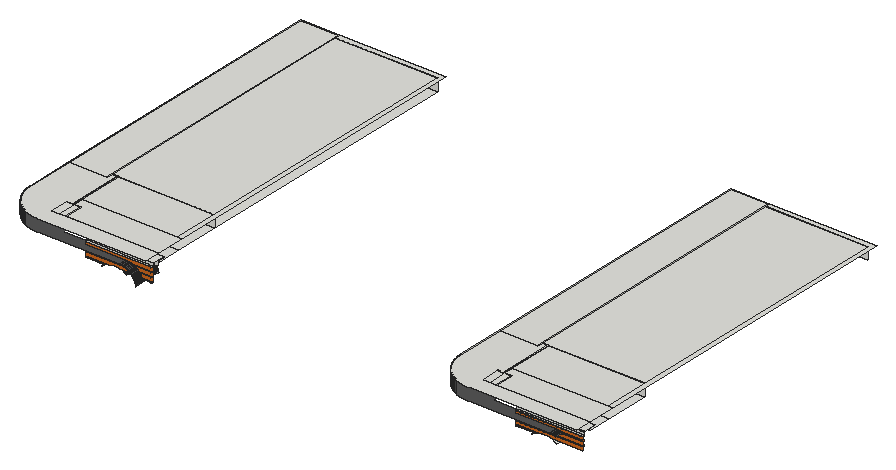
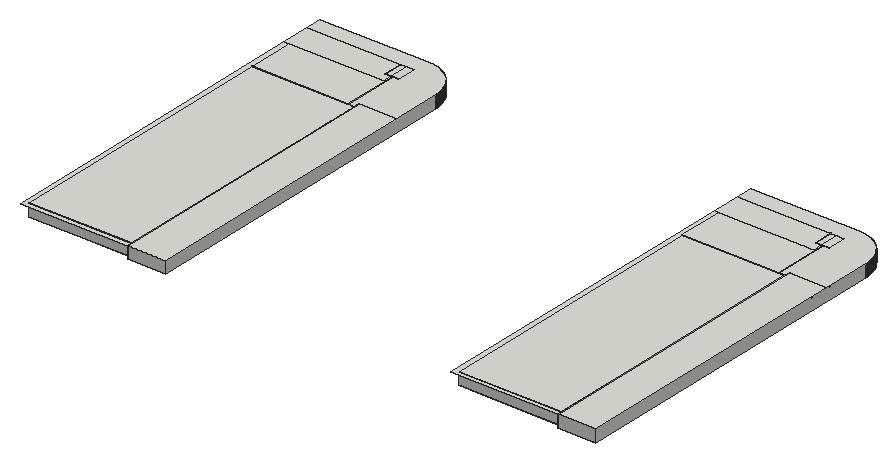
# SketchUp Ruby script. Lengths in inches.
U = 1.inch
M = Sketchup.active_model
def pt(a) = Geom::Point3d.new(a.map { |v| v * U })
def face(e, loops, mat)
  f = e.add_face(loops[0].map { |a| pt(a) })
  loops[1..].each { |l| e.add_face(l.map { |a| pt(a) }).erase! }
  f.material = f.back_material = mat if mat
  f
end
# faces: each face lists its corners as indices into pts; further lists are holes
def faces(e, pts, list, mat = nil) = list.each { |f| face(e, (f[0].is_a?(Array) ? f : [f]).map { |l| l.map { |i| pts[i] } }, mat) }
# xy, xz, yz: faces in a plane at the given z, y or x. An outline is a flat list of corners, or four numbers for a rectangle; further outlines are holes
def ring(l) = l.size == 4 ? [[l[0], l[1]], [l[2], l[1]], [l[2], l[3]], [l[0], l[3]]] : l.each_slice(2).to_a
def flat(e, list, mat, &to3) = list.each { |f| face(e, (f[0].is_a?(Array) ? f : [f]).map { |l| ring(l).map { |u, v| to3.(u, v) } }, mat) }
def xy(e, z, list, mat = nil) = flat(e, list, mat) { |x, y| [x, y, z] }
def xz(e, y, list, mat = nil) = flat(e, list, mat) { |x, z| [x, y, z] }
def yz(e, x, list, mat = nil) = flat(e, list, mat) { |y, z| [x, y, z] }
def lines(e, pts, list) = list.each { |a, b| e.add_line(pt(pts[a]), pt(pts[b])) }
# prism: a flat outline (further loops are holes) pulled along v
def prism(e, loops, v, mat = nil)
  f = face(e, loops, mat); d = Geom::Vector3d.new(v.map { |x| x * U })
  f.pushpull(f.normal.samedirection?(d) ? d.length : -d.length)
end
def box(e, o, s, mat = nil) = prism(e, [[o, [o[0] + s[0], o[1], o[2]], [o[0] + s[0], o[1] + s[1], o[2]], [o[0], o[1] + s[1], o[2]]]], [0, 0, s[2]], mat)
def at(x, y, z, deg = 0) = Geom::Transformation.translation(pt([x, y, z])) * Geom::Transformation.rotation(ORIGIN, Z_AXIS, deg.degrees)
def axes(o, x, y, z) = Geom::Transformation.new([*x, 0, *y, 0, *z, 0, *pt(o).to_a, 1])
def part(name) = M.definitions.add(name)
# library, detail: a bought-in or finely detailed component or shape, given as its bounding box
def library(name, o, s) = part(name).tap { |d| box(d.entities, o, s) }
def detail(e, o, s) = box(e.add_group.entities, o, s)
def put(e, d, t, mat = nil) = e.add_instance(d, t).tap { |i| i.material = mat if mat }
def group(e, t, mat = nil) = e.add_group.tap { |g| g.transformation = t; g.material = mat if mat }.entities
root = M.entities
M.materials.add("[0041_Chocolate]").color = [210, 105, 30]
M.materials.add("[Color M06]").color = [84, 84, 84]
xy(root,385.02,[[820.52,971.36,850.01,972.36],[877.83,971.36,921.96,972.36],[1476.02,971.36,1505.51,972.36]],"[0041_Chocolate]")
xy(root,386.9375,[[820.52,971.36,854.99,972.36],[872.87,971.36,921.96,972.36],[1476.02,971.36,1510.49,972.36]],"[0041_Chocolate]")
xy(root,391.89,[[820.52,971.36,921.96,972.36],[1476.02,971.36,1577.46,972.36]],"[0041_Chocolate]")
xy(root,393.8125,[[820.52,971.36,921.96,972.36],[1476.02,971.36,1577.46,972.36]],"[0041_Chocolate]")
xy(root,395.26,[[820.52,993.35,899.77,1001.16],[1476.02,993.35,1555.27,1001.16]])
xy(root,398.77,[[820.52,971.36,921.96,972.36],[1476.02,971.36,1577.46,972.36]],"[0041_Chocolate]")
xy(root,400.6875,[[820.52,971.36,921.96,972.36],[1476.02,971.36,1577.46,972.36]],"[0041_Chocolate]")
xy(root,402.64,[[820.52,991.23,881.73,993.35],[1476.02,991.23,1537.23,993.35],[913.34,993.35,916.04,993.35,916.04,1028.46,769.03,1028.46,769.03,1012.23,780.56,1012.23,780.56,996.48,820.52,996.48,820.52,1003.71,913.34,1003.71],[820.52,993.35,913.34,1003.71],[1568.84,993.35,1571.54,993.35,1571.54,1028.46,1424.53,1028.46,1424.53,1012.23,1436.06,1012.23,1436.06,996.48,1476.02,996.48,1476.02,1003.71,1568.84,1003.71],
  [1476.02,993.35,1568.84,1003.71],[759.32,996.48,769.03,1003.71],[769.03,996.48,780.56,1003.71],[1414.82,996.48,1424.53,1003.71],[1424.53,996.48,1436.06,1003.71],
  [759.32,1003.71,769.03,1012.23],[769.03,1003.71,780.56,1012.23],[1414.82,1003.71,1424.53,1012.23],[1424.53,1003.71,1436.06,1012.23],[769.03,1028.46,916.04,1097.28],
  [1424.53,1028.46,1571.54,1097.28],[767.84,1089.96,769.03,1097.28],[1423.34,1089.96,1424.53,1097.28],[759.32,1097.28,767.84,1521.81],[767.84,1097.28,879.04,1521.81],
  [879.04,1097.28,916.04,1521.81],[1414.82,1097.28,1423.34,1521.81],[1423.34,1097.28,1534.54,1521.81]])
xy(root,402.64,[[758.26,958.64,756.78,958.66,755.29,958.72,753.8,958.82,752.32,958.96,750.84,959.13,749.37,959.34,747.9,959.6,746.4375,959.89,744.98,960.22,743.54,960.58,742.11,960.99,740.6875,961.43,739.28,961.91,737.88,962.42,736.49,962.97,735.125,963.5625,733.77,964.1875,732.4375,964.84,731.12,965.54,729.82,966.27,728.54,967.03,727.28,967.82,726.04,968.65,724.83,969.51,723.63,970.4,722.46,971.32,721.32,972.27,720.2,973.26,719.11,974.27,718.04,975.31,717,976.37,715.99,977.47,715.01,978.59,714.06,979.73,713.13,980.9,712.24,982.09,711.38,983.31,710.56,984.55,709.76,985.81,709,987.09,708.27,988.39,707.58,989.71,706.92,991.04,706.3,992.39,705.71,993.76,705.16,995.14,704.64,996.54,704.16,997.95,703.72,999.375,703.32,1000.81,702.95,1002.25,702.62,1003.7,702.33,1005.16,702.08,1006.63,701.86,1008.11,701.6875,1009.58,701.55,1011.07,701.46,1012.55,701.4,1014.04,701.38,1015.53,701.38,1529.04,759.32,1529.04,759.32,996.48,780.56,996.48,780.56,978.84,820.52,978.84,820.52,991.23,881.73,991.23,881.73,958.64],[1413.76,958.64,1412.28,958.66,1410.79,958.72,1409.3,958.82,1407.82,958.96,1406.34,959.13,1404.87,959.34,1403.4,959.6,1401.9375,959.89,1400.48,960.22,1399.04,960.58,1397.61,960.99,1396.1875,961.43,1394.78,961.91,1393.38,962.42,1391.99,962.97,1390.625,963.5625,1389.27,964.1875,1387.9375,964.84,1386.62,965.54,1385.32,966.27,1384.04,967.03,1382.78,967.82,1381.54,968.65,1380.33,969.51,1379.13,970.4,1377.96,971.32,1376.82,972.27,1375.7,973.26,1374.61,974.27,1373.54,975.31,1372.5,976.37,1371.49,977.47,1370.51,978.59,1369.56,979.73,1368.63,980.9,1367.74,982.09,1366.88,983.31,1366.06,984.55,1365.26,985.81,1364.5,987.09,1363.77,988.39,1363.08,989.71,1362.42,991.04,1361.8,992.39,1361.21,993.76,1360.66,995.14,1360.14,996.54,1359.66,997.95,1359.22,999.375,1358.82,1000.81,1358.45,1002.25,1358.12,1003.7,1357.83,1005.16,1357.58,1006.63,1357.36,1008.11,1357.1875,1009.58,1357.05,1011.07,1356.96,1012.55,1356.9,1014.04,1356.88,1015.53,1356.88,1529.04,1414.82,1529.04,1414.82,996.48,1436.06,996.48,1436.06,978.84,1476.02,978.84,1476.02,991.23,1537.23,991.23,1537.23,958.64]],"[Color M06]")
xy(root,405.64,[[820.52,971.36,921.96,972.36],[1476.02,971.36,1577.46,972.36]],"[0041_Chocolate]")
xy(root,411.82,[[820.52,972.36,921.96,993.35],[1476.02,972.36,1577.46,993.35]])
xy(root,421.25,[[758.26,958.64,922.83,958.64,922.83,983.34,759.32,983.34,759.32,1012.23,767.84,1012.23,767.84,1097.28,759.32,1097.28,759.32,1088.75,701.38,1088.75,701.38,1015.53,701.4,1014.04,701.46,1012.55,701.55,1011.07,701.6875,1009.58,701.86,1008.11,702.08,1006.63,702.33,1005.16,702.62,1003.7,702.95,1002.25,703.32,1000.81,703.72,999.375,704.16,997.95,704.64,996.54,705.16,995.14,705.71,993.76,706.3,992.39,706.92,991.04,707.58,989.71,708.27,988.39,709,987.09,709.76,985.81,710.56,984.55,711.38,983.31,712.24,982.09,713.13,980.9,714.06,979.73,715.01,978.59,715.99,977.47,717,976.37,718.04,975.31,719.11,974.27,720.2,973.26,721.32,972.27,722.46,971.32,723.63,970.4,724.83,969.51,726.04,968.65,727.28,967.82,728.54,967.03,729.82,966.27,731.12,965.54,732.4375,964.84,733.77,964.1875,735.125,963.5625,736.49,962.97,737.88,962.42,739.28,961.91,740.6875,961.43,742.11,960.99,743.54,960.58,744.98,960.22,746.4375,959.89,747.9,959.6,749.37,959.34,750.84,959.13,752.32,958.96,753.8,958.82,755.29,958.72,756.78,958.66],[1413.76,958.64,1578.33,958.64,1578.33,983.34,1414.82,983.34,1414.82,1012.23,1423.34,1012.23,1423.34,1097.28,1414.82,1097.28,1414.82,1088.75,1356.88,1088.75,1356.88,1015.53,1356.9,1014.04,1356.96,1012.55,1357.05,1011.07,1357.1875,1009.58,1357.36,1008.11,1357.58,1006.63,1357.83,1005.16,1358.12,1003.7,1358.45,1002.25,1358.82,1000.81,1359.22,999.375,1359.66,997.95,1360.14,996.54,1360.66,995.14,1361.21,993.76,1361.8,992.39,1362.42,991.04,1363.08,989.71,1363.77,988.39,1364.5,987.09,1365.26,985.81,1366.06,984.55,1366.88,983.31,1367.74,982.09,1368.63,980.9,1369.56,979.73,1370.51,978.59,1371.49,977.47,1372.5,976.37,1373.54,975.31,1374.61,974.27,1375.7,973.26,1376.82,972.27,1377.96,971.32,1379.13,970.4,1380.33,969.51,1381.54,968.65,1382.78,967.82,1384.04,967.03,1385.32,966.27,1386.62,965.54,1387.9375,964.84,1389.27,964.1875,1390.625,963.5625,1391.99,962.97,1393.38,962.42,1394.78,961.91,1396.1875,961.43,1397.61,960.99,1399.04,960.58,1400.48,960.22,1401.9375,959.89,1403.4,959.6,1404.87,959.34,1406.34,959.13,1407.82,958.96,1409.3,958.82,1410.79,958.72,1412.28,958.66],[759.32,983.34,770.9,1012.23],[770.9,983.34,780.56,1012.23],[780.56,983.34,922.83,983.34,922.83,1027.17,770.9,1027.17,770.9,1012.23,780.56,1012.23],
  [1414.82,983.34,1426.4,1012.23],[1426.4,983.34,1436.06,1012.23],[1436.06,983.34,1578.33,983.34,1578.33,1027.17,1426.4,1027.17,1426.4,1012.23,1436.06,1012.23],[767.84,1012.23,769.03,1097.28],[769.03,1012.23,770.9,1012.23,770.9,1027.17,916.04,1027.17,916.04,1097.28,769.03,1097.28],
  [1423.34,1012.23,1424.53,1097.28],[1424.53,1012.23,1426.4,1012.23,1426.4,1027.17,1571.54,1027.17,1571.54,1097.28,1424.53,1097.28],[916.04,1027.17,922.83,1027.17,922.83,1529.04,759.32,1529.04,759.32,1521.81,916.04,1521.81],[1571.54,1027.17,1578.33,1027.17,1578.33,1529.04,1414.82,1529.04,1414.82,1521.81,1571.54,1521.81],[701.38,1088.75,759.32,1529.04],
  [1356.88,1088.75,1414.82,1529.04],[759.32,1097.28,916.04,1521.81],[1414.82,1097.28,1571.54,1521.81]])
xz(root,971.36,[[820.52,386.9375,854.99,386.9375,859.81,388.23,868,388.24,872.87,386.9375,921.96,386.9375,921.96,391.89,820.52,391.89],[1476.02,386.9375,1510.49,386.9375,1515.31,388.23,1523.5,388.24,1528.37,386.9375,1577.46,386.9375,1577.46,391.89,1476.02,391.89],[820.52,393.8125,921.96,398.77],[1476.02,393.8125,1577.46,398.77],[820.52,400.6875,921.96,405.64],
  [1476.02,400.6875,1577.46,405.64]],"[0041_Chocolate]")
xz(root,972.36,[[820.52,405.64,921.96,407.5625],[1476.02,405.64,1577.46,407.5625],[820.52,407.5625,921.96,411.82],[1476.02,407.5625,1577.46,411.82],[820.52,411.82,921.96,412.52],
  [1476.02,411.82,1577.46,412.52]])
xz(root,972.36,[[820.52,385.02,850.01,385.02,851.91,386.11,854.99,386.9375,820.52,386.9375],[877.83,385.02,921.96,385.02,921.96,386.9375,872.87,386.9375,875.91,386.125],[1476.02,385.02,1505.51,385.02,1507.41,386.11,1510.49,386.9375,1476.02,386.9375],[820.52,391.89,921.96,393.8125],[1476.02,391.89,1577.46,393.8125],
  [820.52,398.77,921.96,400.6875],[1476.02,398.77,1577.46,400.6875]],"[0041_Chocolate]")
xz(root,993.35,[[820.52,395.26,899.77,395.26,899.46,395.5625,898.97,396.02,898.46,396.46,897.94,396.89,897.41,397.3125,896.87,397.72,896.32,398.1,895.76,398.48,895.19,398.84,894.61,399.18,894.02,399.51,893.43,399.83,892.82,400.125,892.21,400.41,891.59,400.67,890.96,400.92,890.33,401.16,889.69,401.375,889.05,401.57,888.4,401.76,887.75,401.92,887.09,402.07,886.43,402.2,885.76,402.32,885.09,402.41,884.42,402.49,883.75,402.56,883.08,402.6,882.41,402.625,881.73,402.64,820.52,402.64],[899.77,395.26,907.49,395.26,907.49,402.64,881.73,402.64,882.41,402.625,883.08,402.6,883.75,402.56,884.42,402.49,885.09,402.41,885.76,402.32,886.43,402.2,887.09,402.07,887.75,401.92,888.4,401.76,889.05,401.57,889.69,401.375,890.33,401.16,890.96,400.92,891.59,400.67,892.21,400.41,892.82,400.125,893.43,399.83,894.02,399.51,894.61,399.18,895.19,398.84,895.76,398.48,896.32,398.1,896.87,397.72,897.41,397.3125,897.94,396.89,898.46,396.46,898.97,396.02,899.46,395.5625],[907.49,395.26,913.34,402.64],[1476.02,395.26,1555.27,395.26,1554.96,395.5625,1554.47,396.02,1553.96,396.46,1553.44,396.89,1552.91,397.3125,1552.37,397.72,1551.82,398.1,1551.26,398.48,1550.69,398.84,1550.11,399.18,1549.52,399.51,1548.93,399.83,1548.32,400.125,1547.71,400.41,1547.09,400.67,1546.46,400.92,1545.83,401.16,1545.19,401.375,1544.55,401.57,1543.9,401.76,1543.25,401.92,1542.59,402.07,1541.93,402.2,1541.26,402.32,1540.59,402.41,1539.92,402.49,1539.25,402.56,1538.58,402.6,1537.91,402.625,1537.23,402.64,1476.02,402.64],[820.52,402.64,907.49,411.82],
  [1476.02,402.64,1562.99,411.82]])
xz(root,1012.23,[[759.32,402.64,767.84,421.25],[767.84,402.64,769.03,421.25],[769.03,402.64,770.9,421.25],[770.9,402.64,780.56,421.25],[1414.82,402.64,1423.34,421.25],
  [1423.34,402.64,1424.53,421.25],[1424.53,402.64,1426.4,421.25],[1426.4,402.64,1436.06,421.25]])
xz(root,1097.28,[[759.32,402.64,767.84,421.25],[767.84,402.64,769.03,421.25],[769.03,402.64,916.04,421.25],[1414.82,402.64,1423.34,421.25],[1423.34,402.64,1424.53,421.25],
  [1424.53,402.64,1571.54,421.25]])
xz(root,1521.81,[[759.32,402.64,916.04,421.25],[1414.82,402.64,1571.54,421.25]])
xz(root,1529.04,[[701.38,402.64,759.32,421.25],[1356.88,402.64,1414.82,421.25]])
yz(root,701.38,[[1015.53,402.64,1529.04,421.25]])
yz(root,759.32,[[1088.75,402.64,1097.28,421.25],[1097.28,402.64,1521.81,421.25],[1521.81,402.64,1529.04,421.25]])
yz(root,769.03,[[1012.23,402.64,1097.28,421.25]])
yz(root,780.56,[[983.34,402.64,1012.23,421.25]])
yz(root,820.52,[[991.23,395.26,993.35,402.64],[993.35,395.26,996.48,402.64]])
yz(root,1356.88,[[1015.53,402.64,1529.04,421.25]])
yz(root,1414.82,[[1088.75,402.64,1097.28,421.25],[1097.28,402.64,1521.81,421.25],[1521.81,402.64,1529.04,421.25]])
yz(root,1424.53,[[1012.23,402.64,1097.28,421.25]])
yz(root,1436.06,[[983.34,402.64,1012.23,421.25]])
yz(root,1476.02,[[991.23,395.26,993.35,402.64],[993.35,395.26,996.48,402.64]])
p = [[907.06,958.64,381.57],[907.06,993.35,381.57],[907.17,993.35,380.9],[907.17,958.64,380.9],[907.17,1001.16,380.9],[907.06,1001.16,381.57],
  [906.93,958.64,382.23],[906.93,993.35,382.23],[906.93,1001.16,382.23],[850.01,986.55,385.02],[850.01,972.36,385.02],[850.01,971.36,385.02],
  [844.82,971.36,382.01],[844.82,986.55,382.01],[883,986.55,382.03],[883,971.36,382.03],[877.83,971.36,385.02],[877.83,972.36,385.02],
  [877.83,986.55,385.02],[1505.51,986.55,385.02],[1505.51,972.36,385.02],[1505.51,971.36,385.02],[1500.32,971.36,382.01],[1500.32,986.55,382.01],
  [1538.5,986.55,382.03],[1538.5,971.36,382.03],[1533.33,971.36,385.02],[1533.33,972.36,385.02],[1533.33,986.55,385.02],[906.78,958.64,382.89],
  [906.78,993.35,382.89],[906.78,1001.16,382.89],[906.61,958.64,383.54],[906.61,993.35,383.54],[906.61,1001.16,383.54],[906.43,958.64,384.19],
  [906.43,993.35,384.19],[906.59,993.35,383.64],[906.59,1001.16,383.64],[906.43,1001.16,384.19],[906.23,958.64,384.84],[906.23,993.35,384.84],
  [906.23,1001.16,384.84],[906.01,958.64,385.47],[906.01,993.35,385.47],[906.01,1001.16,385.47],[851.91,972.36,386.11],[851.91,986.55,386.11],
  [875.91,972.36,386.125],[875.91,986.55,386.125],[1507.41,972.36,386.11],[1507.41,986.55,386.11],[1531.41,972.36,386.125],[1531.41,986.55,386.125],
  [905.78,958.64,386.11],[905.78,993.35,386.11],[905.91,993.35,385.76],[905.91,1001.16,385.76],[905.78,1001.16,386.11],[905.53,958.64,386.73],
  [905.53,993.35,386.73],[854.99,972.36,386.9375],[854.99,986.55,386.9375],[872.87,972.36,386.9375],[872.87,986.55,386.9375],[1510.49,972.36,386.9375],
  [1510.49,986.55,386.9375],[1528.37,972.36,386.9375],[1528.37,986.55,386.9375],[905.53,1001.16,386.73],[905.26,958.64,387.35],[905.26,993.35,387.35],
  [905.26,1001.16,387.35],[859.81,986.55,388.23],[859.81,971.36,388.23],[854.99,971.36,386.9375],[872.87,971.36,386.9375],[868,971.36,388.24],
  [868,986.55,388.24],[1515.31,986.55,388.23],[1515.31,971.36,388.23],[1510.49,971.36,386.9375],[1528.37,971.36,386.9375],[1523.5,971.36,388.24],
  [1523.5,986.55,388.24],[904.98,958.64,387.96],[904.98,993.35,387.96],[904.98,1001.16,387.96],[904.68,958.64,388.57],[904.68,993.35,388.57],
  [904.68,1001.16,388.57],[904.37,958.64,389.17],[904.37,993.35,389.17],[904.37,1001.16,389.17],[904.04,958.64,389.76],[904.04,993.35,389.76],
  [904.04,1001.16,389.76],[903.7,958.64,390.33],[903.7,993.35,390.33],[903.7,1001.16,390.33],[903.34,958.64,390.9],[903.34,993.35,390.9],
  [903.34,1001.16,390.9],[902.96,958.64,391.47],[902.96,993.35,391.47],[902.96,1001.16,391.47],[902.57,958.64,392.02],[902.57,993.35,392.02],
  [902.57,1001.16,392.02],[902.17,958.64,392.56],[902.17,993.35,392.56],[902.17,1001.16,392.56],[901.75,958.64,393.09],[901.75,993.35,393.09],
  [901.75,1001.16,393.09],[901.32,958.64,393.6],[901.32,993.35,393.6],[901.71,993.35,393.14],[901.71,1001.16,393.14],[901.32,1001.16,393.6],
  [900.875,958.64,394.11],[900.875,993.35,394.11],[900.875,1001.16,394.11],[900.42,958.64,394.61],[900.42,993.35,394.61],[900.42,1001.16,394.61],
  [899.95,958.64,395.09],[899.95,993.35,395.09],[899.95,1001.16,395.09],[899.46,958.64,395.5625],[899.46,991.23,395.5625],[899.77,991.23,395.26],
  [899.77,993.35,395.26],[899.77,1001.16,395.26],[899.46,993.35,395.5625],[898.97,958.64,396.02],[898.97,991.23,396.02],[898.97,993.35,396.02],
  [898.46,958.64,396.46],[898.46,991.23,396.46],[898.46,993.35,396.46],[897.94,958.64,396.89],[897.94,991.23,396.89],[897.94,993.35,396.89],
  [897.41,958.64,397.3125],[897.41,991.23,397.3125],[897.41,993.35,397.3125],[896.87,958.64,397.72],[896.87,991.23,397.72],[896.87,993.35,397.72],
  [896.32,958.64,398.1],[896.32,991.23,398.1],[896.32,993.35,398.1],[895.76,958.64,398.48],[895.76,991.23,398.48],[895.76,993.35,398.48],
  [895.19,958.64,398.84],[895.19,991.23,398.84],[895.19,993.35,398.84],[894.61,958.64,399.18],[894.61,991.23,399.18],[894.61,993.35,399.18],
  [894.02,958.64,399.51],[894.02,991.23,399.51],[894.02,993.35,399.51],[893.43,958.64,399.83],[893.43,991.23,399.83],[893.43,993.35,399.83],
  [892.82,958.64,400.125],[892.82,991.23,400.125],[892.82,993.35,400.125],[892.21,958.64,400.41],[892.21,991.23,400.41],[892.21,993.35,400.41],
  [891.59,958.64,400.67],[891.59,991.23,400.67],[891.59,993.35,400.67],[890.96,958.64,400.92],[890.96,991.23,400.92],[1546.46,958.64,400.92],
  [1546.46,991.23,400.92],[1547.09,991.23,400.67],[1547.09,958.64,400.67],[890.96,993.35,400.92],[1546.46,993.35,400.92],[1547.09,993.35,400.67],
  [890.33,958.64,401.16],[890.33,991.23,401.16],[1545.83,958.64,401.16],[1545.83,991.23,401.16],[890.33,993.35,401.16],[1545.83,993.35,401.16],
  [889.69,958.64,401.375],[889.69,991.23,401.375],[1545.19,958.64,401.375],[1545.19,991.23,401.375],[889.69,993.35,401.375],[1545.19,993.35,401.375],
  [889.05,958.64,401.57],[889.05,991.23,401.57],[1544.55,958.64,401.57],[1544.55,991.23,401.57],[889.05,993.35,401.57],[1544.55,993.35,401.57],
  [888.4,958.64,401.76],[888.4,991.23,401.76],[1543.9,958.64,401.76],[1543.9,991.23,401.76],[888.4,993.35,401.76],[1543.9,993.35,401.76],
  [887.75,958.64,401.92],[887.75,991.23,401.92],[1543.25,958.64,401.92],[1543.25,991.23,401.92],[887.75,993.35,401.92],[1543.25,993.35,401.92],
  [887.09,958.64,402.07],[887.09,991.23,402.07],[1542.59,958.64,402.07],[1542.59,991.23,402.07],[887.09,993.35,402.07],[1542.59,993.35,402.07],
  [886.43,958.64,402.2],[886.43,991.23,402.2],[1541.93,958.64,402.2],[1541.93,991.23,402.2],[886.43,993.35,402.2],[1541.93,993.35,402.2],
  [885.76,958.64,402.32],[885.76,991.23,402.32],[1541.26,958.64,402.32],[1541.26,991.23,402.32],[885.76,993.35,402.32],[1541.26,993.35,402.32],
  [885.09,958.64,402.41],[885.09,991.23,402.41],[1540.59,958.64,402.41],[1540.59,991.23,402.41],[885.09,993.35,402.41],[1540.59,993.35,402.41],
  [884.42,958.64,402.49],[884.42,991.23,402.49],[1539.92,958.64,402.49],[1539.92,991.23,402.49],[884.42,993.35,402.49],[1539.92,993.35,402.49],
  [883.75,958.64,402.56],[883.75,991.23,402.56],[1539.25,958.64,402.56],[1539.25,991.23,402.56],[883.75,993.35,402.56],[1539.25,993.35,402.56],
  [881.73,958.64,402.64],[881.73,991.23,402.64],[882.41,991.23,402.625],[882.41,958.64,402.625],[883.08,991.23,402.6],[883.08,958.64,402.6],
  [1537.23,958.64,402.64],[1537.23,991.23,402.64],[1537.91,991.23,402.625],[1537.91,958.64,402.625],[1538.58,991.23,402.6],[1538.58,958.64,402.6],
  [733.77,964.1875,421.25],[732.4375,964.84,421.25],[732.4375,964.84,402.64],[733.77,964.1875,402.64],[1389.27,964.1875,421.25],[1387.9375,964.84,421.25],
  [1387.9375,964.84,402.64],[1389.27,964.1875,402.64],[731.12,965.54,421.25],[731.12,965.54,402.64],[1386.62,965.54,421.25],[1386.62,965.54,402.64],
  [729.82,966.27,421.25],[729.82,966.27,402.64],[1385.32,966.27,421.25],[1385.32,966.27,402.64],[728.54,967.03,421.25],[728.54,967.03,402.64],
  [1384.04,967.03,421.25],[1384.04,967.03,402.64],[727.28,967.82,421.25],[727.28,967.82,402.64],[1382.78,967.82,421.25],[1382.78,967.82,402.64],
  [726.04,968.65,421.25],[726.04,968.65,402.64],[1381.54,968.65,421.25],[1381.54,968.65,402.64],[724.83,969.51,421.25],[724.83,969.51,402.64],
  [1380.33,969.51,421.25],[1380.33,969.51,402.64],[723.63,970.4,421.25],[723.63,970.4,402.64],[1379.13,970.4,421.25],[1379.13,970.4,402.64],
  [722.46,971.32,421.25],[722.46,971.32,402.64],[1377.96,971.32,421.25],[1377.96,971.32,402.64],[721.32,972.27,421.25],[721.32,972.27,402.64],
  [1376.82,972.27,421.25],[1376.82,972.27,402.64],[720.2,973.26,421.25],[720.2,973.26,402.64],[1375.7,973.26,421.25],[1375.7,973.26,402.64],
  [719.11,974.27,421.25],[719.11,974.27,402.64],[1374.61,974.27,421.25],[1374.61,974.27,402.64],[718.04,975.31,421.25],[718.04,975.31,402.64],
  [1373.54,975.31,421.25],[1373.54,975.31,402.64],[717,976.37,421.25],[717,976.37,402.64],[1372.5,976.37,421.25],[1372.5,976.37,402.64],
  [715.99,977.47,421.25],[715.99,977.47,402.64],[1371.49,977.47,421.25],[1371.49,977.47,402.64],[715.01,978.59,421.25],[715.01,978.59,402.64],
  [1370.51,978.59,421.25],[1370.51,978.59,402.64],[714.06,979.73,421.25],[714.06,979.73,402.64],[1369.56,979.73,421.25],[1369.56,979.73,402.64],
  [713.13,980.9,421.25],[713.13,980.9,402.64],[1368.63,980.9,421.25],[1368.63,980.9,402.64],[712.24,982.09,421.25],[712.24,982.09,402.64],
  [1367.74,982.09,421.25],[1367.74,982.09,402.64],[711.38,983.31,421.25],[711.38,983.31,402.64],[1366.88,983.31,421.25],[1366.88,983.31,402.64],
  [710.56,984.55,421.25],[710.56,984.55,402.64],[1366.06,984.55,421.25],[1366.06,984.55,402.64],[709.76,985.81,421.25],[709.76,985.81,402.64],
  [1365.26,985.81,421.25],[1365.26,985.81,402.64],[709,987.09,421.25],[709,987.09,402.64],[1364.5,987.09,421.25],[1364.5,987.09,402.64],
  [708.27,988.39,421.25],[708.27,988.39,402.64],[1363.77,988.39,421.25],[1363.77,988.39,402.64],[707.58,989.71,421.25],[707.58,989.71,402.64],
  [1363.08,989.71,421.25],[1363.08,989.71,402.64],[706.92,991.04,421.25],[706.92,991.04,402.64],[1362.42,991.04,421.25],[1362.42,991.04,402.64],
  [706.3,992.39,421.25],[706.3,992.39,402.64],[1361.8,992.39,421.25],[1361.8,992.39,402.64],[881.73,993.35,402.64],[882.41,993.35,402.625],
  [883.08,993.35,402.6],[1537.23,993.35,402.64],[1537.91,993.35,402.625],[1538.58,993.35,402.6],[705.71,993.76,421.25],[705.71,993.76,402.64],
  [1361.21,993.76,421.25],[1361.21,993.76,402.64],[705.16,995.14,421.25],[705.16,995.14,402.64],[1360.66,995.14,421.25],[1360.66,995.14,402.64],
  [704.64,996.54,421.25],[704.64,996.54,402.64],[1360.14,996.54,421.25],[1360.14,996.54,402.64],[704.16,997.95,421.25],[704.16,997.95,402.64],
  [1359.66,997.95,421.25],[1359.66,997.95,402.64],[703.72,999.375,421.25],[703.72,999.375,402.64],[1359.22,999.375,421.25],[1359.22,999.375,402.64],
  [703.32,1000.81,421.25],[703.32,1000.81,402.64],[1358.82,1000.81,421.25],[1358.82,1000.81,402.64],[702.95,1002.25,421.25],[702.95,1002.25,402.64],
  [1358.45,1002.25,421.25],[1358.45,1002.25,402.64],[702.62,1003.7,421.25],[702.62,1003.7,402.64],[1358.12,1003.7,421.25],[1358.12,1003.7,402.64],
  [702.33,1005.16,421.25],[702.33,1005.16,402.64],[1357.83,1005.16,421.25],[1357.83,1005.16,402.64],[702.08,1006.63,421.25],[702.08,1006.63,402.64],
  [1357.58,1006.63,421.25],[1357.58,1006.63,402.64],[701.86,1008.11,421.25],[701.86,1008.11,402.64],[1357.36,1008.11,421.25],[1357.36,1008.11,402.64],
  [701.6875,1009.58,421.25],[701.6875,1009.58,402.64],[1357.1875,1009.58,421.25],[1357.1875,1009.58,402.64],[701.55,1011.07,421.25],[701.55,1011.07,402.64],
  [1357.05,1011.07,421.25],[1357.05,1011.07,402.64],[701.46,1012.55,421.25],[701.46,1012.55,402.64],[1356.96,1012.55,421.25],[1356.96,1012.55,402.64],
  [701.4,1014.04,421.25],[701.4,1014.04,402.64],[1356.9,1014.04,421.25],[1356.9,1014.04,402.64],[701.38,1015.53,421.25],[701.38,1015.53,402.64],
  [1356.88,1015.53,421.25],[1356.88,1015.53,402.64]]
faces(root,p,[[0,1,2,3],[6,7,1,0],[29,30,7,6],[32,33,30,29],[35,36,37,33,32],[40,41,36,35],[43,44,41,40],[54,55,56,44,43],
  [59,60,55,54],[70,71,60,59],[85,86,71,70],[88,89,86,85],[91,92,89,88],[94,95,92,91],[97,98,95,94],[100,101,98,97],
  [103,104,101,100],[106,107,104,103],[109,110,107,106],[112,113,110,109],[115,116,117,113,112],[120,121,116,115],[123,124,121,120],[126,127,124,123],
  [129,130,131,132,127,126],[135,136,130,129],[138,139,136,135],[141,142,139,138],[144,145,142,141],[147,148,145,144],[150,151,148,147],[153,154,151,150],
  [156,157,154,153],[159,160,157,156],[162,163,160,159],[165,166,163,162],[168,169,166,165],[171,172,169,168],[174,175,172,171],[177,178,175,174],
  [179,180,181,182],[186,187,178,177],[188,189,180,179],[192,193,187,186],[194,195,189,188],[198,199,193,192],[200,201,195,194],[204,205,199,198],
  [206,207,201,200],[210,211,205,204],[212,213,207,206],[216,217,211,210],[218,219,213,212],[222,223,217,216],[224,225,219,218],[228,229,223,222],
  [230,231,225,224],[234,235,229,228],[236,237,231,230],[240,241,235,234],[242,243,237,236],[246,247,241,240],[248,249,243,242],[252,253,254,255],
  [255,254,256,257],[257,256,247,246],[258,259,260,261],[261,260,262,263],[263,262,249,248],[264,265,266,267],[268,269,270,271],[265,272,273,266],
  [269,274,275,270],[272,276,277,273],[274,278,279,275],[276,280,281,277],[278,282,283,279],[280,284,285,281],[282,286,287,283],[284,288,289,285],
  [286,290,291,287],[288,292,293,289],[290,294,295,291],[292,296,297,293],[294,298,299,295],[296,300,301,297],[298,302,303,299],[300,304,305,301],
  [302,306,307,303],[304,308,309,305],[306,310,311,307],[308,312,313,309],[310,314,315,311],[312,316,317,313],[314,318,319,315],[316,320,321,317],
  [318,322,323,319],[320,324,325,321],[322,326,327,323],[324,328,329,325],[326,330,331,327],[328,332,333,329],[330,334,335,331],[332,336,337,333],
  [334,338,339,335],[336,340,341,337],[338,342,343,339],[340,344,345,341],[342,346,347,343],[344,348,349,345],[346,350,351,347],[348,352,353,349],
  [350,354,355,351],[352,356,357,353],[354,358,359,355],[356,360,361,357],[358,362,363,359],[360,364,365,361],[362,366,367,363],[364,368,369,365],
  [366,370,371,367],[368,372,373,369],[370,374,375,371],[372,382,383,373],[374,384,385,375],[382,386,387,383],[384,388,389,385],[386,390,391,387],
  [388,392,393,389],[390,394,395,391],[392,396,397,393],[394,398,399,395],[396,400,401,397],[398,402,403,399],[400,404,405,401],[402,406,407,403],
  [404,408,409,405],[406,410,411,407],[408,412,413,409],[410,414,415,411],[412,416,417,413],[414,418,419,415],[416,420,421,417],[418,422,423,419],
  [420,424,425,421],[422,426,427,423],[424,428,429,425],[426,430,431,427],[428,432,433,429],[430,434,435,431],[432,436,437,433],[434,438,439,435],
  [436,440,441,437],[438,442,443,439],[440,444,445,441]],"[Color M06]")
faces(root,p,[[1,2,4,5],[7,1,5,8],[9,10,11,12,13],[14,15,16,17,18],[19,20,21,22,23],[24,25,26,27,28],[30,7,8,31],[33,30,31,34],
  [37,33,34,38],[36,37,38,39],[41,36,39,42],[44,41,42,45],[46,10,9,47],[17,48,49,18],[50,20,19,51],[27,52,53,28],
  [56,44,45,57],[55,56,57,58],[61,46,47,62],[48,63,64,49],[65,50,51,66],[52,67,68,53],[60,55,58,69],[71,60,69,72],
  [73,74,75,61,62],[64,63,76,77,78],[79,80,81,65,66],[68,67,82,83,84],[86,71,72,87],[89,86,87,90],[78,77,74,73],[84,83,80,79],
  [92,89,90,93],[95,92,93,96],[98,95,96,99],[101,98,99,102],[104,101,102,105],[107,104,105,108],[110,107,108,111],[113,110,111,114],
  [116,117,118,119],[117,113,114,118],[121,116,119,122],[124,121,122,125],[127,124,125,128],[132,127,128,133],[134,132,131,130],[137,134,130,136],
  [140,137,136,139],[143,140,139,142],[146,143,142,145],[149,146,145,148],[152,149,148,151],[155,152,151,154],[158,155,154,157],[161,158,157,160],
  [164,161,160,163],[167,164,163,166],[170,167,166,169],[173,170,169,172],[176,173,172,175],[183,176,175,178],[184,185,181,180],[190,183,178,187],
  [191,184,180,189],[196,190,187,193],[197,191,189,195],[202,196,193,199],[203,197,195,201],[208,202,199,205],[209,203,201,207],[214,208,205,211],
  [215,209,207,213],[220,214,211,217],[221,215,213,219],[226,220,217,223],[227,221,219,225],[232,226,223,229],[233,227,225,231],[238,232,229,235],
  [239,233,231,237],[244,238,235,241],[245,239,237,243],[250,244,241,247],[251,245,243,249],[376,377,254,253],[377,378,256,254],[378,250,247,256],
  [379,380,260,259],[380,381,262,260],[381,251,249,262]])
